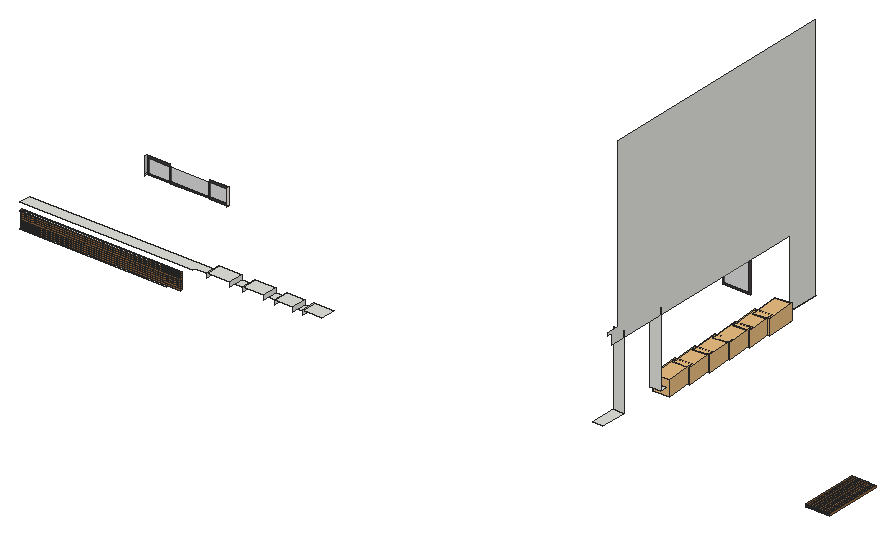
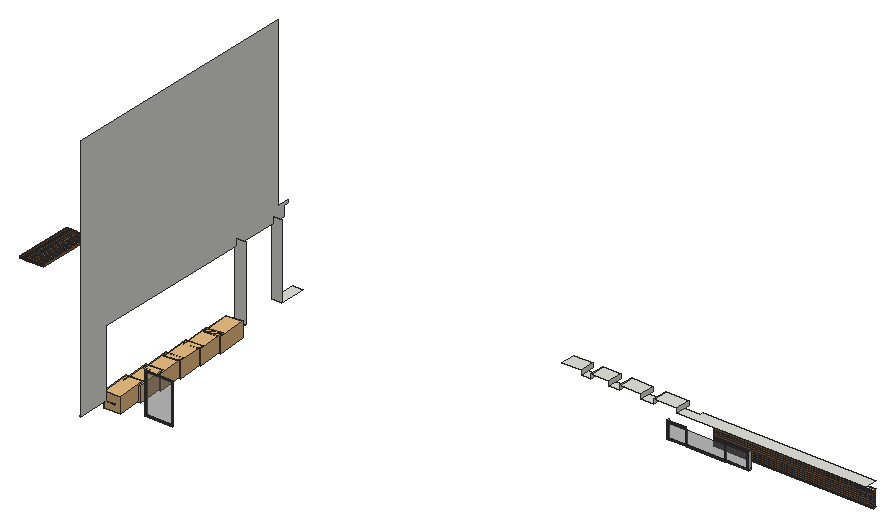
# SketchUp Ruby script. Lengths in inches.
U = 1.inch
M = Sketchup.active_model
def pt(a) = Geom::Point3d.new(a.map { |v| v * U })
def face(e, loops, mat)
  f = e.add_face(loops[0].map { |a| pt(a) })
  loops[1..].each { |l| e.add_face(l.map { |a| pt(a) }).erase! }
  f.material = f.back_material = mat if mat
  f
end
# faces: each face lists its corners as indices into pts; further lists are holes
def faces(e, pts, list, mat = nil) = list.each { |f| face(e, (f[0].is_a?(Array) ? f : [f]).map { |l| l.map { |i| pts[i] } }, mat) }
# xy, xz, yz: faces in a plane at the given z, y or x. An outline is a flat list of corners, or four numbers for a rectangle; further outlines are holes
def ring(l) = l.size == 4 ? [[l[0], l[1]], [l[2], l[1]], [l[2], l[3]], [l[0], l[3]]] : l.each_slice(2).to_a
def flat(e, list, mat, &to3) = list.each { |f| face(e, (f[0].is_a?(Array) ? f : [f]).map { |l| ring(l).map { |u, v| to3.(u, v) } }, mat) }
def xy(e, z, list, mat = nil) = flat(e, list, mat) { |x, y| [x, y, z] }
def xz(e, y, list, mat = nil) = flat(e, list, mat) { |x, z| [x, y, z] }
def yz(e, x, list, mat = nil) = flat(e, list, mat) { |y, z| [x, y, z] }
def lines(e, pts, list) = list.each { |a, b| e.add_line(pt(pts[a]), pt(pts[b])) }
# prism: a flat outline (further loops are holes) pulled along v
def prism(e, loops, v, mat = nil)
  f = face(e, loops, mat); d = Geom::Vector3d.new(v.map { |x| x * U })
  f.pushpull(f.normal.samedirection?(d) ? d.length : -d.length)
end
def box(e, o, s, mat = nil) = prism(e, [[o, [o[0] + s[0], o[1], o[2]], [o[0] + s[0], o[1] + s[1], o[2]], [o[0], o[1] + s[1], o[2]]]], [0, 0, s[2]], mat)
def at(x, y, z, deg = 0) = Geom::Transformation.translation(pt([x, y, z])) * Geom::Transformation.rotation(ORIGIN, Z_AXIS, deg.degrees)
def axes(o, x, y, z) = Geom::Transformation.new([*x, 0, *y, 0, *z, 0, *pt(o).to_a, 1])
def part(name) = M.definitions.add(name)
# library, detail: a bought-in or finely detailed component or shape, given as its bounding box
def library(name, o, s) = part(name).tap { |d| box(d.entities, o, s) }
def detail(e, o, s) = box(e.add_group.entities, o, s)
def put(e, d, t, mat = nil) = e.add_instance(d, t).tap { |i| i.material = mat if mat }
def group(e, t, mat = nil) = e.add_group.tap { |g| g.transformation = t; g.material = mat if mat }.entities
root = M.entities
M.materials.add("[0009_Linen]").color = [250, 240, 230]
M.materials.add("[Asphalt New]").color = [67, 60, 62]
M.materials.add("[Polished Concrete New]").color = [200, 200, 203]
M.materials.add("[Translucent Glass Gray]").color = [128, 128, 128]
M.materials["[Translucent Glass Gray]"].alpha = 0.5
M.materials.add("[Wood Floor]").color = [155, 105, 61]
c1 = part("Group\#2")
xy(c1.entities,0,[[0,0,1.85,1.85],[2.64,0,4.49,1.85],[5.28,0,7.125,1.85],[7.91,0,9.76,1.85],[10.55,0,12.4,1.85],
  [13.1875,0,15.04,1.85],[15.83,0,17.68,1.85],[18.46,0,20.31,1.85],[21.1,0,22.95,1.85]],"[Wood Floor]")
g1 = group(c1.entities,at(0,0,0))
xy(g1,112.2,[[0,0,1.85,1.85],[2.64,0,4.49,1.85],[5.28,0,7.125,1.85],[7.91,0,9.76,1.85],[10.55,0,12.4,1.85],
  [13.1875,0,15.04,1.85],[15.83,0,17.68,1.85],[18.46,0,20.31,1.85],[21.1,0,22.95,1.85]],"[Wood Floor]")
xz(g1,0,[[0,0,1.85,112.2],[2.64,0,4.49,112.2],[5.28,0,7.125,112.2],[7.91,0,9.76,112.2],[10.55,0,12.4,112.2],
  [13.1875,0,15.04,112.2],[15.83,0,17.68,112.2],[18.46,0,20.31,112.2],[21.1,0,22.95,112.2]],"[Wood Floor]")
xz(g1,1.85,[[0,0,1.85,112.2],[2.64,0,4.49,112.2],[5.28,0,7.125,112.2],[7.91,0,9.76,112.2],[10.55,0,12.4,112.2],
  [13.1875,0,15.04,112.2],[15.83,0,17.68,112.2],[18.46,0,20.31,112.2],[21.1,0,22.95,112.2]],"[Wood Floor]")
yz(g1,0,[[0,0,1.85,112.2]],"[Wood Floor]")
yz(g1,1.85,[[0,0,1.85,112.2]],"[Wood Floor]")
yz(g1,2.64,[[0,0,1.85,112.2]],"[Wood Floor]")
yz(g1,4.49,[[0,0,1.85,112.2]],"[Wood Floor]")
yz(g1,5.28,[[0,0,1.85,112.2]],"[Wood Floor]")
yz(g1,7.125,[[0,0,1.85,112.2]],"[Wood Floor]")
yz(g1,7.91,[[0,0,1.85,112.2]],"[Wood Floor]")
yz(g1,9.76,[[0,0,1.85,112.2]],"[Wood Floor]")
yz(g1,10.55,[[0,0,1.85,112.2]],"[Wood Floor]")
yz(g1,12.4,[[0,0,1.85,112.2]],"[Wood Floor]")
yz(g1,13.1875,[[0,0,1.85,112.2]],"[Wood Floor]")
yz(g1,15.04,[[0,0,1.85,112.2]],"[Wood Floor]")
yz(g1,15.83,[[0,0,1.85,112.2]],"[Wood Floor]")
yz(g1,17.68,[[0,0,1.85,112.2]],"[Wood Floor]")
yz(g1,18.46,[[0,0,1.85,112.2]],"[Wood Floor]")
yz(g1,20.31,[[0,0,1.85,112.2]],"[Wood Floor]")
yz(g1,21.1,[[0,0,1.85,112.2]],"[Wood Floor]")
yz(g1,22.95,[[0,0,1.85,112.2]],"[Wood Floor]")
c2 = library("Plante \#58",[-0.43,-1.58,0],[20.84,18.06,17.59])
xy(root,97.93,[[20.0625,153.99,321.78,160.36]])
xy(root,119.9375,[[1155.46,203.31,1176.625,256.56],[1155.46,349.72,1176.625,349.72,1176.625,747.375,1174.71,747.375,1174.71,683.93,1155.46,683.93]])
xy(root,131.1875,[[20.0625,153.99,347.76,160.36]])
xy(root,146.4375,[[20.0625,153.99,373.77,153.99,373.77,160.36,408.3,160.36,408.3,178.37,20.0625,178.37],[454.65,160.36,481.51,178.37],[525.01,160.36,547.38,178.37],[584.28,160.36,603.91,178.37]])
xy(root,155.375,[[408.3,148.8,454.65,178.37],[481.51,148.8,525.01,178.37],[547.38,148.8,584.28,178.37],[603.91,148.8,643.56,178.37]])
xz(root,256.56,[[1155.46,119.9375,1176.625,272.3125]])
xz(root,304.24,[[160.07,181.51,164.29,184.14],[164.29,181.51,208.29,184.14],[208.29,181.51,210.23,184.14],[210.23,181.51,286.57,184.14],[286.57,181.51,288.77,184.14],
  [288.77,181.51,323.93,184.14],[323.93,181.51,328.15,184.14],[160.07,184.14,164.29,184.14,164.29,212.5,208.29,212.5,208.29,216.73,160.07,216.73],[208.29,184.14,210.23,212.5],[286.57,184.14,288.77,212.5],
  [323.93,184.14,328.15,184.14,328.15,216.73,288.77,216.73,288.77,212.5,323.93,212.5]],"[Asphalt New]")
xz(root,304.24,[[164.29,184.14,208.29,212.5],[210.23,184.14,286.57,212.5],[288.77,184.14,323.93,212.5]],"[Translucent Glass Gray]")
xz(root,349.72,[[1155.46,119.9375,1176.625,272.3125]])
xz(root,683.93,[[[1036.79,120.97,1094.73,206.28],[1039.99,124.17,1091.52,203.07]]],"[Asphalt New]")
xz(root,683.93,[[1039.99,124.17,1091.52,203.07]],"[Translucent Glass Gray]")
yz(root,160.07,[[298.43,181.51,304.24,184.14],[298.43,184.14,304.24,216.73]],"[Polished Concrete New]")
yz(root,328.15,[[300.43,181.51,304.24,184.14],[300.43,184.14,304.24,216.73]],"[0009_Linen]")
yz(root,408.3,[[148.8,146.4375,178.37,155.375]])
yz(root,454.65,[[148.8,146.4375,178.37,155.375]])
yz(root,481.51,[[148.8,146.4375,178.37,155.375]])
yz(root,525.01,[[148.8,146.4375,178.37,155.375]])
yz(root,547.38,[[148.8,146.4375,178.37,155.375]])
yz(root,584.28,[[148.8,146.4375,178.37,155.375]])
yz(root,603.91,[[148.8,146.4375,178.37,155.375]])
yz(root,1174.71,[[683.93,119.9375,747.375,119.9375,747.375,626.3125,242.24,626.3125,242.24,285.125,216.68,285.125,216.68,278.88,228.43,278.88,228.43,258.1,683.93,258.1]])
put(root,c1,axes([1560.35,243.73,93.37],[2.12,0,0],[0,0,-2.12],[0,1.04732,0]))
put(root,c1,axes([347.76,156.4375,97.93],[0,0,1.44909],[0,2.12,0],[-2.92049,0,0]))
put(root,c2,axes([1147.77,629.67,104.16],[0.24325,-2.99012,0],[1.82397,0.14838,0],[0,0,1.785]))
put(root,c2,axes([1147.77,578.67,104.16],[0.24325,-2.99012,0],[1.82397,0.14838,0],[0,0,1.785]))
put(root,c2,axes([1147.77,527.67,104.16],[0.24325,-2.99012,0],[1.82397,0.14838,0],[0,0,1.785]))
put(root,c2,axes([1147.77,476.67,104.16],[0.24325,-2.99012,0],[1.82397,0.14838,0],[0,0,1.785]))
put(root,c2,axes([1147.77,425.67,104.16],[0.24325,-2.99012,0],[1.82397,0.14838,0],[0,0,1.785]))
put(root,c2,axes([1149.64,678.4,105],[0.24325,-2.99012,0],[1.82397,0.14838,0],[0,0,1.785]))
